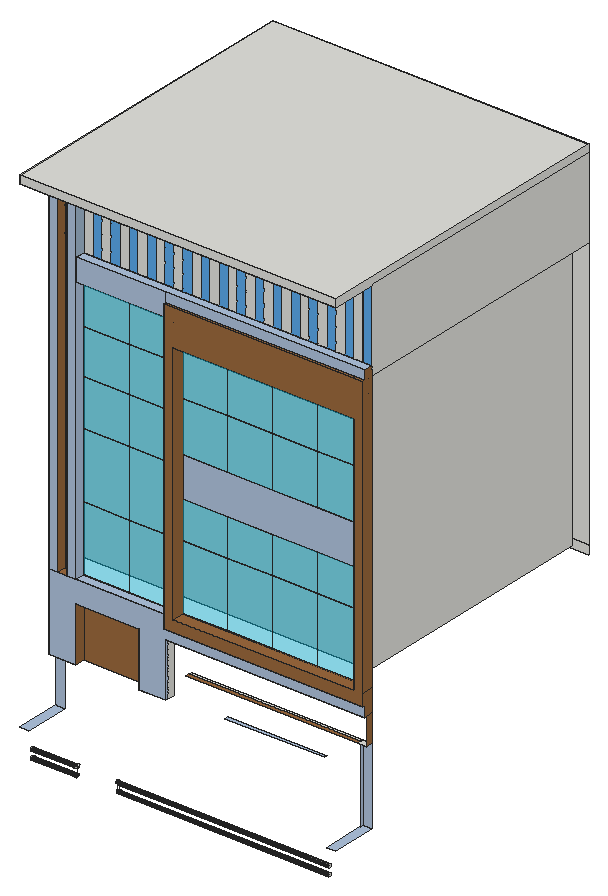
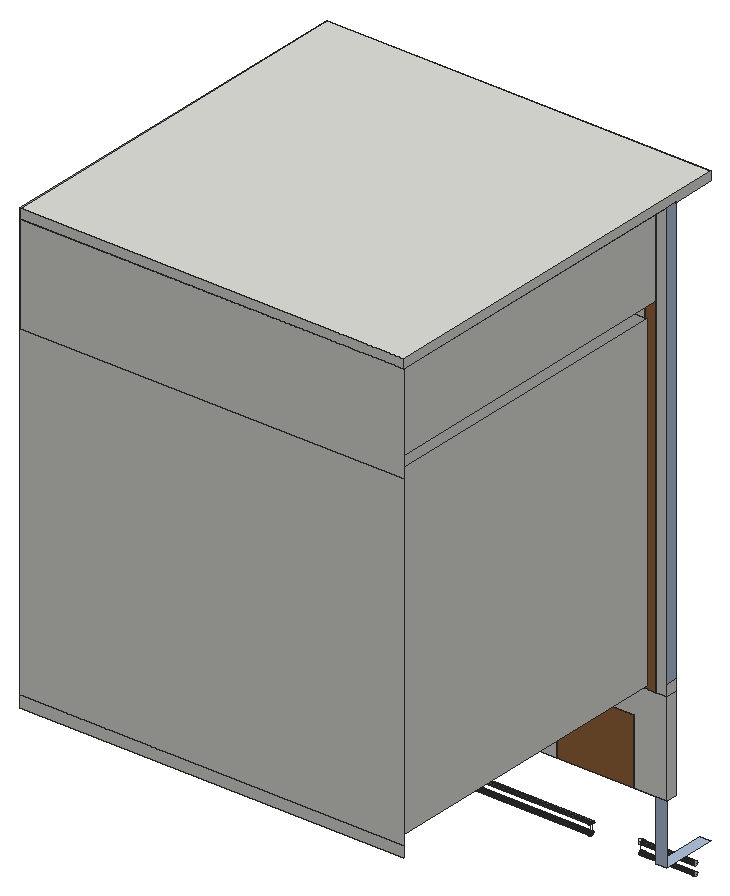
# SketchUp Ruby script. Lengths in inches.
U = 1.inch
M = Sketchup.active_model
def pt(a) = Geom::Point3d.new(a.map { |v| v * U })
def face(e, loops, mat)
  f = e.add_face(loops[0].map { |a| pt(a) })
  loops[1..].each { |l| e.add_face(l.map { |a| pt(a) }).erase! }
  f.material = f.back_material = mat if mat
  f
end
# faces: each face lists its corners as indices into pts; further lists are holes
def faces(e, pts, list, mat = nil) = list.each { |f| face(e, (f[0].is_a?(Array) ? f : [f]).map { |l| l.map { |i| pts[i] } }, mat) }
# xy, xz, yz: faces in a plane at the given z, y or x. An outline is a flat list of corners, or four numbers for a rectangle; further outlines are holes
def ring(l) = l.size == 4 ? [[l[0], l[1]], [l[2], l[1]], [l[2], l[3]], [l[0], l[3]]] : l.each_slice(2).to_a
def flat(e, list, mat, &to3) = list.each { |f| face(e, (f[0].is_a?(Array) ? f : [f]).map { |l| ring(l).map { |u, v| to3.(u, v) } }, mat) }
def xy(e, z, list, mat = nil) = flat(e, list, mat) { |x, y| [x, y, z] }
def xz(e, y, list, mat = nil) = flat(e, list, mat) { |x, z| [x, y, z] }
def yz(e, x, list, mat = nil) = flat(e, list, mat) { |y, z| [x, y, z] }
def lines(e, pts, list) = list.each { |a, b| e.add_line(pt(pts[a]), pt(pts[b])) }
# prism: a flat outline (further loops are holes) pulled along v
def prism(e, loops, v, mat = nil)
  f = face(e, loops, mat); d = Geom::Vector3d.new(v.map { |x| x * U })
  f.pushpull(f.normal.samedirection?(d) ? d.length : -d.length)
end
def box(e, o, s, mat = nil) = prism(e, [[o, [o[0] + s[0], o[1], o[2]], [o[0] + s[0], o[1] + s[1], o[2]], [o[0], o[1] + s[1], o[2]]]], [0, 0, s[2]], mat)
def at(x, y, z, deg = 0) = Geom::Transformation.translation(pt([x, y, z])) * Geom::Transformation.rotation(ORIGIN, Z_AXIS, deg.degrees)
def axes(o, x, y, z) = Geom::Transformation.new([*x, 0, *y, 0, *z, 0, *pt(o).to_a, 1])
def part(name) = M.definitions.add(name)
# library, detail: a bought-in or finely detailed component or shape, given as its bounding box
def library(name, o, s) = part(name).tap { |d| box(d.entities, o, s) }
def detail(e, o, s) = box(e.add_group.entities, o, s)
def put(e, d, t, mat = nil) = e.add_instance(d, t).tap { |i| i.material = mat if mat }
def group(e, t, mat = nil) = e.add_group.tap { |g| g.transformation = t; g.material = mat if mat }.entities
root = M.entities
M.materials.add("[0099_LightSteelBlue]").color = [176, 196, 222]
M.materials.add("[0100_SteelBlue]").color = [91, 169, 234]
M.materials.add("[0110_LightSlateGray]").color = [164, 188, 211]
M.materials.add("[Metal Corrugated Shiny]").color = [124, 124, 124]
M.materials.add("[Translucent Glass Tinted]").color = [8, 201, 241]
M.materials["[Translucent Glass Tinted]"].alpha = 0.48
M.materials.add("[Wood Floor]").color = [155, 105, 61]
xy(root,151.31,[[126.03,62.85,126.54,62.97,126.99,63.22,127.37,63.58,127.64,64.02,127.79,64.52,127.8,64.83,127.8,65.05,127.68,65.55,127.43,66.01,127.07,66.39,126.625,66.66,126.125,66.81,125.6,66.82,125.1,66.7,124.64,66.45,124.26,66.09,123.99,65.64,123.84,65.14,123.83,64.62,123.95,64.11,124.2,63.66,124.56,63.28,125.01,63.01,125.51,62.86]])
xy(root,153,[[72.44,62.83,72.96,62.9,73.44,63.1,73.86,63.42,74.17,63.83,74.375,64.32,74.44,64.83,74.375,65.35,74.17,65.83,73.86,66.25,73.44,66.57,72.96,66.77,72.44,66.83,71.92,66.77,71.44,66.57,71.03,66.25,70.71,65.83,70.51,65.35,70.44,64.83,70.51,64.32,70.71,63.83,71.03,63.42,71.44,63.1,71.92,62.9]])
xy(root,175,[[0,60,12,120],[408,60,420,120]],"[0099_LightSteelBlue]")
xy(root,241,[[0,108,12,120],[12,108,36,120],[120,108,156,120],[228,116,360,120]],"[0099_LightSteelBlue]")
xy(root,277,[[408,111,420,120],[180,116,408,120]])
xy(root,277,[[180,111,408,116]],"[Wood Floor]")
xy(root,313,[[156,111,420,120]])
xy(root,313,[[156,108,420,111]],"[0099_LightSteelBlue]")
xy(root,313,[[36,108,120,120]],"[Wood Floor]")
xy(root,328,[[156,104,420,108]],"[Wood Floor]")
xy(root,343,[[167.5,104,168,108],[408,104,420,120],[0,108,12,120],[24,108,36,120],[167.5,108,168,120]])
xy(root,343,[[36,108,167.5,120]],"[0099_LightSteelBlue]")
xy(root,343,[[168,104,408,120],[12,108,24,120]],"[Wood Floor]")
xy(root,355,[[12,132,408,468]])
xy(root,667,[[167.5,104,168,108],[156,108,167.5,120],[167.5,108,168,120],[201.43,110.45,200.65,110.5,199.91,110.76,199.26,111.2,198.75,111.79,198.41,112.5,198.26,113.27,198.32,114.05,198.58,114.79,199.02,115.44,199.61,115.95,200.3125,116.29,201.08,116.4375,201.86,116.38,202.6,116.12,203.25,115.68,203.76,115.09,204.11,114.39,204.25,113.62,204.2,112.84,203.9375,112.1,203.5,111.45,202.91,110.94,202.2,110.59],[261.5,110.45,260.71,110.5,259.97,110.76,259.33,111.2,258.8125,111.79,258.47,112.5,258.33,113.27,258.38,114.05,258.64,114.79,259.08,115.44,259.67,115.95,260.375,116.29,261.15,116.4375,261.93,116.38,262.67,116.12,263.3125,115.68,263.83,115.09,264.17,114.39,264.32,113.62,264.26,112.84,264,112.1,263.5625,111.45,262.97,110.94,262.26,110.59],
  [323.56,110.45,322.78,110.5,322.04,110.76,321.39,111.2,320.875,111.79,320.54,112.5,320.39,113.27,320.44,114.05,320.7,114.79,321.14,115.44,321.73,115.95,322.4375,116.29,323.21,116.4375,323.99,116.38,324.73,116.12,325.375,115.68,325.89,115.09,326.23,114.39,326.38,113.62,326.32,112.84,326.0625,112.1,325.625,111.45,325.03,110.94,324.33,110.59],[380.12,110.45,379.34,110.5,378.6,110.76,377.95,111.2,377.4375,111.79,377.1,112.5,376.95,113.27,377.01,114.05,377.26,114.79,377.7,115.44,378.3,115.95,379,116.29,379.77,116.4375,380.55,116.38,381.29,116.12,381.9375,115.68,382.45,115.09,382.79,114.39,382.94,113.62,382.88,112.84,382.625,112.1,382.1875,111.45,381.59,110.94,380.89,110.59]])
xy(root,667,[[[168,104,408,120],[261.5,110.45,262.26,110.59,262.97,110.94,263.5625,111.45,264,112.1,264.26,112.84,264.32,113.62,264.17,114.39,263.83,115.09,263.3125,115.68,262.67,116.12,261.93,116.38,261.15,116.4375,260.375,116.29,259.67,115.95,259.08,115.44,258.64,114.79,258.38,114.05,258.33,113.27,258.47,112.5,258.8125,111.79,259.33,111.2,259.97,110.76,260.71,110.5],[323.56,110.45,324.33,110.59,325.03,110.94,325.625,111.45,326.0625,112.1,326.32,112.84,326.38,113.62,326.23,114.39,325.89,115.09,325.375,115.68,324.73,116.12,323.99,116.38,323.21,116.4375,322.4375,116.29,321.73,115.95,321.14,115.44,320.7,114.79,320.44,114.05,320.39,113.27,320.54,112.5,320.875,111.79,321.39,111.2,322.04,110.76,322.78,110.5],[380.12,110.45,380.89,110.59,381.59,110.94,382.1875,111.45,382.625,112.1,382.88,112.84,382.94,113.62,382.79,114.39,382.45,115.09,381.9375,115.68,381.29,116.12,380.55,116.38,379.77,116.4375,379,116.29,378.3,115.95,377.7,115.44,377.26,114.79,377.01,114.05,376.95,113.27,377.1,112.5,377.4375,111.79,377.95,111.2,378.6,110.76,379.34,110.5],[201.43,110.45,202.2,110.59,202.91,110.94,203.5,111.45,203.9375,112.1,204.2,112.84,204.25,113.62,204.11,114.39,203.76,115.09,203.25,115.68,202.6,116.12,201.86,116.38,201.08,116.4375,200.3125,116.29,199.61,115.95,199.02,115.44,198.58,114.79,198.32,114.05,198.26,113.27,198.41,112.5,198.75,111.79,199.26,111.2,199.91,110.76,200.65,110.5]]],"[Wood Floor]")
xy(root,697,[[36,108,156,120],[156,108,168,120]])
xy(root,715,[[156,104,408,108],[408,104,420,108]],"[Wood Floor]")
xy(root,727,[[36,108,420,120]],"[0099_LightSteelBlue]")
xy(root,822.5,[[12,120,408,468]])
xy(root,822.6875,[[82.7,87.46,81.41,87.61,80.2,88.1,79.15,88.88,78.34,89.91,77.83,91.11,77.64,92.4,77.8,93.69,78.28,94.91,79.0625,95.95,80.09,96.76,81.29,97.27,82.58,97.46,83.875,97.3,85.09,96.82,86.13,96.04,86.94,95.01,87.46,93.8125,87.64,92.52,87.49,91.23,87,90.01,86.22,88.97,85.2,88.16,84,87.65],[149.39,87.46,148.1,87.61,146.88,88.1,145.84,88.88,145.03,89.91,144.52,91.11,144.33,92.4,144.48,93.69,144.97,94.91,145.75,95.95,146.78,96.76,147.98,97.27,149.27,97.46,150.5625,97.3,151.78,96.82,152.82,96.04,153.63,95.01,154.14,93.8125,154.33,92.52,154.17,91.23,153.69,90.01,152.91,88.97,151.88,88.16,150.68,87.65],[227.64,87.46,226.35,87.61,225.13,88.1,224.09,88.88,223.28,89.91,222.77,91.11,222.58,92.4,222.73,93.69,223.22,94.91,224,95.95,225.03,96.76,226.23,97.27,227.52,97.46,228.8125,97.3,230.03,96.82,231.07,96.04,231.88,95.01,232.39,93.8125,232.58,92.52,232.42,91.23,231.94,90.01,231.16,88.97,230.13,88.16,228.93,87.65],[312.95,87.46,311.66,87.61,310.45,88.1,309.4,88.88,308.59,89.91,308.08,91.11,307.89,92.4,308.05,93.69,308.53,94.91,309.3125,95.95,310.34,96.76,311.54,97.27,312.83,97.46,314.125,97.3,315.34,96.82,316.38,96.04,317.19,95.01,317.71,93.8125,317.89,92.52,317.74,91.23,317.25,90.01,316.47,88.97,315.45,88.16,314.25,87.65]])
xy(root,822.6875,[[[0,60,0,108,12,108,12,120,24,120,24,108,36,108,36,120,420,120,420,60],[312.95,87.46,314.25,87.65,315.45,88.16,316.47,88.97,317.25,90.01,317.74,91.23,317.89,92.52,317.71,93.8125,317.19,95.01,316.38,96.04,315.34,96.82,314.125,97.3,312.83,97.46,311.54,97.27,310.34,96.76,309.3125,95.95,308.53,94.91,308.05,93.69,307.89,92.4,308.08,91.11,308.59,89.91,309.4,88.88,310.45,88.1,311.66,87.61],[149.39,87.46,150.68,87.65,151.88,88.16,152.91,88.97,153.69,90.01,154.17,91.23,154.33,92.52,154.14,93.8125,153.63,95.01,152.82,96.04,151.78,96.82,150.5625,97.3,149.27,97.46,147.98,97.27,146.78,96.76,145.75,95.95,144.97,94.91,144.48,93.69,144.33,92.4,144.52,91.11,145.03,89.91,145.84,88.88,146.88,88.1,148.1,87.61],[227.64,87.46,228.93,87.65,230.13,88.16,231.16,88.97,231.94,90.01,232.42,91.23,232.58,92.52,232.39,93.8125,231.88,95.01,231.07,96.04,230.03,96.82,228.8125,97.3,227.52,97.46,226.23,97.27,225.03,96.76,224,95.95,223.22,94.91,222.73,93.69,222.58,92.4,222.77,91.11,223.28,89.91,224.09,88.88,225.13,88.1,226.35,87.61],[82.7,87.46,84,87.65,85.2,88.16,86.22,88.97,87,90.01,87.49,91.23,87.64,92.52,87.46,93.8125,86.94,95.01,86.13,96.04,85.09,96.82,83.875,97.3,82.58,97.46,81.29,97.27,80.09,96.76,79.0625,95.95,78.28,94.91,77.8,93.69,77.64,92.4,77.83,91.11,78.34,89.91,79.15,88.88,80.2,88.1,81.41,87.61]]],"[0100_SteelBlue]")
xy(root,823,[[0,108,12,120],[24,108,36,120],[0,120,0,480,420,480,420,120,408,120,408,468,12,468,12,120],[12,120,408,468]])
xy(root,833,[[0,60,420,480]])
xz(root,60,[[0,822.6875,420,833]])
xz(root,104,[[156,328,420,328,420,343,167.5,343,167.5,667,408,667,408,343,420,343,420,715,156,715],[167.5,343,168,667]],"[Wood Floor]")
xz(root,108,[[156,667,168,697],[0,822.6875,12,823],[24,822.6875,36,823]])
xz(root,108,[[0,241,36,241,36,313,120,313,120,241,156,241,156,313,420,313,420,328,156,328,156,343,0,343],[0,343,12,822.6875],[24,343,36,822.6875],[36,697,156,727],[156,715,420,727]],"[0099_LightSteelBlue]")
xz(root,120,[[0,241,0,343,420,343,420,313,156,313,156,241,120,241,120,313,36,313,36,241],[0,343,12,823],[24,343,36,727],[167.5,343,168,667],[408,343,420,355],
  [408,355,420,697],[168,667,168,697,36,697,36,727,420,727,420,697,408,697,408,667],[156,667,168,697],[24,727,36,822.5],[36,727,48,822.5],
  [60,727,72,822.5],[84,727,96,822.5],[108,727,120,822.5],[132,727,144,822.5],[156,727,168,822.5],
  [180,727,192,822.5],[204,727,216,822.5],[228,727,240,822.5],[252,727,264,822.5],[276,727,288,822.5],
  [300,727,312,822.5],[324,727,336,822.5],[348,727,360,822.5],[372,727,384,822.5],[396,727,408,822.5],
  [12,822.5,24,822.6875],[24,822.5,36,823],[36,822.5,48,822.6875],[48,822.5,60,822.6875],[60,822.5,72,822.6875],
  [72,822.5,84,822.6875],[84,822.5,96,822.6875],[96,822.5,108,822.6875],[108,822.5,120,822.6875],[120,822.5,132,822.6875],
  [132,822.5,144,822.6875],[144,822.5,156,822.6875],[156,822.5,168,822.6875],[168,822.5,180,822.6875],[180,822.5,192,822.6875],
  [192,822.5,204,822.6875],[204,822.5,216,822.6875],[216,822.5,228,822.6875],[228,822.5,240,822.6875],[240,822.5,252,822.6875],
  [252,822.5,264,822.6875],[264,822.5,276,822.6875],[276,822.5,288,822.6875],[288,822.5,300,822.6875],[300,822.5,312,822.6875],
  [312,822.5,324,822.6875],[324,822.5,336,822.6875],[336,822.5,348,822.6875],[348,822.5,360,822.6875],[360,822.5,372,822.6875],
  [372,822.5,384,822.6875],[384,822.5,396,822.6875],[396,822.5,408,822.6875],[12,822.6875,24,823],[36,822.6875,48,823],
  [48,822.6875,60,823],[60,822.6875,72,823],[72,822.6875,84,823],[84,822.6875,96,823],[96,822.6875,108,823],
  [108,822.6875,120,823],[120,822.6875,132,823],[132,822.6875,144,823],[144,822.6875,156,823],[156,822.6875,168,823],
  [168,822.6875,180,823],[180,822.6875,192,823],[192,822.6875,204,823],[204,822.6875,216,823],[216,822.6875,228,823],
  [228,822.6875,240,823],[240,822.6875,252,823],[252,822.6875,264,823],[264,822.6875,276,823],[276,822.6875,288,823],
  [288,822.6875,300,823],[300,822.6875,312,823],[312,822.6875,324,823],[324,822.6875,336,823],[336,822.6875,348,823],
  [348,822.6875,360,823],[360,822.6875,372,823],[372,822.6875,384,823],[384,822.6875,396,823],[396,822.6875,408,823],
  [408,822.6875,420,823]])
xz(root,120,[[0,175,12,241],[408,175,420,277],[168,479.27,408,531.9]],"[0099_LightSteelBlue]")
xz(root,120,[[48,727,60,822.5],[72,727,84,822.5],[96,727,108,822.5],[120,727,132,822.5],[144,727,156,822.5],
  [168,727,180,822.5],[192,727,204,822.5],[216,727,228,822.5],[240,727,252,822.5],[264,727,276,822.5],
  [288,727,300,822.5],[312,727,324,822.5],[336,727,348,822.5],[360,727,372,822.5],[384,727,396,822.5],
  [408,727,420,822.6875]],"[0100_SteelBlue]")
xz(root,120,[[36,343,98.3125,429.625],[98.3125,343,167.5,429.625],[168,343,228,429.625],[228,343,288,429.625],[288,343,348,429.625],
  [348,343,408,429.625],[36,429.625,98.3125,516.6875],[98.3125,429.625,167.5,516.6875],[168,429.625,228,479.27],[228,429.625,288,479.27],
  [288,429.625,348,479.27],[348,429.625,408,479.27],[36,516.6875,98.3125,578.8125],[98.3125,516.6875,167.5,578.8125],[168,531.9,228,599.25],
  [228,531.9,288,599.25],[288,531.9,348,599.25],[348,531.9,408,599.25],[36,578.8125,98.3125,638.75],[98.3125,578.8125,167.5,638.75],
  [168,599.25,228,667],[228,599.25,288,667],[288,599.25,348,667],[348,599.25,408,667],[36,638.75,98.3125,697],
  [98.3125,638.75,167.5,638.75,167.5,667,156,667,156,697,98.3125,697]],"[Translucent Glass Tinted]")
xz(root,120,[[36,241,120,313],[12,343,24,822.5]],"[Wood Floor]")
xz(root,132,[[12,355,408,715]])
xz(root,468,[[12,355,408,715],[12,727,408,822.5],[12,822.5,408,823]])
xz(root,480,[[0,343,420,355],[0,355,420,715],[0,715,420,823],[0,823,420,833]])
yz(root,0,[[108,241,120,343],[108,343,120,355],[60,822.6875,60,833,480,833,480,823,108,823,108,822.6875]])
yz(root,0,[[108,355,120,823]],"[0099_LightSteelBlue]")
yz(root,12,[[64.83,138.5625,64.32,138.63,63.83,138.83,63.42,139.15,63.1,139.5625,62.9,140.05,62.83,140.5625,62.9,141.08,63.1,141.5625,63.42,141.98,63.83,142.3,64.32,142.5,64.83,142.5625,65.35,142.5,65.83,142.3,66.25,141.98,66.57,141.5625,66.77,141.08,66.83,140.5625,66.77,140.05,66.57,139.5625,66.25,139.15,65.83,138.83,65.35,138.63],[64.83,149.25,64.32,149.32,63.83,149.52,63.42,149.84,63.1,150.25,62.9,150.73,62.83,151.25,62.9,151.77,63.1,152.25,63.42,152.67,63.83,152.98,64.32,153.18,64.83,153.25,65.35,153.18,65.83,152.98,66.25,152.67,66.57,152.25,66.77,151.77,66.83,151.25,66.77,150.73,66.57,150.25,66.25,149.84,65.83,149.52,65.35,149.32],[132,355,468,715],[120,727,468,822.5],[120,822.5,468,823],
  [108,822.6875,120,823]])
yz(root,12,[[108,343,120,822.6875]],"[Wood Floor]")
yz(root,24,[[108,822.6875,120,823]])
yz(root,24,[[108,343,120,822.6875]],"[Wood Floor]")
yz(root,36,[[108,697,120,727],[108,822.6875,120,823]])
yz(root,36,[[108,343,120,697]],"[0099_LightSteelBlue]")
yz(root,36,[[108,727,120,822.6875]],"[0110_LightSlateGray]")
yz(root,36,[[108,241,120,313]],"[Wood Floor]")
yz(root,70.8125,[[64.83,149.25,65.35,149.32,65.83,149.52,66.25,149.84,66.57,150.25,66.77,150.73,66.83,151.25,66.77,151.77,66.57,152.25,66.25,152.67,65.83,152.98,65.35,153.18,64.83,153.25,64.32,153.18,63.83,152.98,63.42,152.67,63.1,152.25,62.9,151.77,62.83,151.25,62.9,150.73,63.1,150.25,63.42,149.84,63.83,149.52,64.32,149.32]])
yz(root,74.44,[[64.83,151.26,64.84,151.27,64.83,151.27]],"[Metal Corrugated Shiny]")
yz(root,120,[[108,241,120,313]],"[Wood Floor]")
yz(root,156,[[111,241,120,313],[104,328,108,343],[108,667,120,697]])
yz(root,156,[[108,241,111,313]],"[0099_LightSteelBlue]")
yz(root,156,[[104,343,108,697],[104,697,108,715]],"[Wood Floor]")
yz(root,167.5,[[104,343,120,667]],"[Wood Floor]")
yz(root,168,[[108,667,120,697]])
yz(root,168,[[104,343,120,667]],"[Wood Floor]")
yz(root,408,[[64.83,138.5625,65.35,138.63,65.83,138.83,66.25,139.15,66.57,139.5625,66.77,140.05,66.83,140.5625,66.77,141.08,66.57,141.5625,66.25,141.98,65.83,142.3,65.35,142.5,64.83,142.5625,64.32,142.5,63.83,142.3,63.42,141.98,63.1,141.5625,62.9,141.08,62.83,140.5625,62.9,140.05,63.1,139.5625,63.42,139.15,63.83,138.83,64.32,138.63],[64.83,149.25,65.35,149.32,65.83,149.52,66.25,149.84,66.57,150.25,66.77,150.73,66.83,151.25,66.77,151.77,66.57,152.25,66.25,152.67,65.83,152.98,65.35,153.18,64.83,153.25,64.32,153.18,63.83,152.98,63.42,152.67,63.1,152.25,62.9,151.77,62.83,151.25,62.9,150.73,63.1,150.25,63.42,149.84,63.83,149.52,64.32,149.32],[132,355,468,715],[114,667,120,697],[120,727,468,822.5],
  [120,822.5,468,823]])
yz(root,408,[[116,175,120,277]],"[0099_LightSteelBlue]")
yz(root,408,[[104,343,120,667]],"[Wood Floor]")
yz(root,420,[[120,715,480,823],[60,822.6875,120,822.6875,120,823,480,823,480,833,60,833]])
yz(root,420,[[111,277,120,313],[108,313,120,313,120,343,104,343,104,328,108,328],[104,343,120,343,120,727,108,727,108,715,104,715]],"[Wood Floor]")
p = [[12,63.83,138.83],[12,64.32,138.63],[70.51,64.32,138.63],[72.44,64.32,138.63],[72.44,63.83,138.83],[70.71,63.83,138.83],
  [408,64.32,138.63],[408,63.83,138.83],[125.82,63.83,138.83],[125.82,64.32,138.63],[12,64.83,138.5625],[70.44,64.83,138.5625],
  [72.44,64.83,138.5625],[408,64.83,138.5625],[125.82,64.83,138.5625],[127.8,64.83,138.5625],[12,65.35,138.63],[70.51,65.35,138.63],
  [72.44,65.35,138.63],[408,65.35,138.63],[125.82,65.35,138.63],[12,65.83,138.83],[70.71,65.83,138.83],[72.44,65.83,138.83],
  [408,65.83,138.83],[125.82,65.83,138.83],[12,63.42,139.15],[72.44,63.42,139.15],[71.03,63.42,139.15],[408,63.42,139.15],
  [125.82,63.42,139.15],[12,66.25,139.15],[71.03,66.25,139.15],[72.44,66.25,139.15],[408,66.25,139.15],[125.82,66.25,139.15],
  [12,63.1,139.5625],[72.44,63.1,139.5625],[71.44,63.1,139.5625],[408,63.1,139.5625],[125.82,63.1,139.5625],[12,66.57,139.5625],
  [71.44,66.57,139.5625],[72.44,66.57,139.5625],[408,66.57,139.5625],[125.82,66.57,139.5625],[12,62.9,140.05],[72.44,62.9,140.05],
  [71.92,62.9,140.05],[408,62.9,140.05],[125.82,62.9,140.05],[12,66.77,140.05],[71.92,66.77,140.05],[72.44,66.77,140.05],
  [408,66.77,140.05],[125.82,66.77,140.05],[12,62.83,140.5625],[72.44,62.83,140.5625],[408,62.83,140.5625],[125.82,62.83,140.5625],
  [12,66.83,140.5625],[72.44,66.83,140.5625],[408,66.83,140.5625],[125.82,66.83,140.5625],[12,62.9,141.08],[72.44,62.9,141.08],
  [71.92,62.9,141.08],[408,62.9,141.08],[125.82,62.9,141.08],[12,66.77,141.08],[71.92,66.77,141.08],[72.44,66.77,141.08],
  [408,66.77,141.08],[125.82,66.77,141.08],[12,63.1,141.5625],[72.44,63.1,141.5625],[71.44,63.1,141.5625],[408,63.1,141.5625],
  [125.82,63.1,141.5625],[12,66.57,141.5625],[71.44,66.57,141.5625],[72.44,66.57,141.5625],[408,66.57,141.5625],[125.82,66.57,141.5625],
  [12,63.42,141.98],[72.44,63.42,141.98],[71.03,63.42,141.98],[408,63.42,141.98],[125.82,63.42,141.98],[12,66.25,141.98],
  [71.03,66.25,141.98],[72.44,66.25,141.98],[408,66.25,141.98],[125.82,66.25,141.98],[12,63.83,142.3],[72.44,63.83,142.3],
  [70.71,63.83,142.3],[408,63.83,142.3],[125.82,63.83,142.3],[12,65.83,142.3],[70.71,65.83,142.3],[72.44,65.83,142.3],
  [408,65.83,142.3],[125.82,65.83,142.3],[12,64.32,142.5],[72.44,64.32,142.5],[70.51,64.32,142.5],[408,64.32,142.5],
  [125.82,64.32,142.5],[12,65.35,142.5],[70.51,65.35,142.5],[72.44,65.35,142.5],[408,65.35,142.5],[125.82,65.35,142.5],
  [12,64.83,142.5625],[72.44,64.83,142.5625],[70.44,64.83,142.5625],[408,64.83,142.5625],[127.8,64.83,142.5625],[125.82,64.83,142.5625],
  [12,63.83,149.52],[12,64.32,149.32],[70.51,64.32,149.32],[70.8125,64.32,149.32],[70.8125,63.83,149.52],[70.71,63.83,149.52],
  [408,64.32,149.32],[408,63.83,149.52],[127.83,63.83,149.52],[127.65,64.32,149.32],[12,64.83,149.25],[70.44,64.83,149.25],
  [70.8125,64.83,149.25],[408,64.83,149.25],[127.33,64.83,149.25],[127.8,64.83,149.25],[12,65.35,149.32],[70.51,65.35,149.32],
  [70.8125,65.35,149.32],[408,65.35,149.32],[126.92,65.35,149.32],[12,65.83,149.52],[70.71,65.83,149.52],[70.8125,65.83,149.52],
  [408,65.83,149.52],[126.43,65.83,149.52],[12,63.42,149.84],[70.8125,63.42,149.84],[408,63.42,149.84],[127.88,63.42,149.84],
  [12,66.25,149.84],[70.8125,66.25,149.84],[408,66.25,149.84],[125.9,66.25,149.84],[12,63.1,150.25],[70.8125,63.1,150.25],
  [408,63.1,150.25],[127.79,63.1,150.25],[12,66.57,150.25],[70.8125,66.57,150.25],[408,66.57,150.25],[125.36,66.57,150.25],
  [73.45,66.12,150.09],[72.96,66.26,149.95],[72.45,66.31,149.9],[71.93,66.26,149.95],[71.45,66.11,150.08],[71.03,65.875,150.29],
  [70.71,65.57,150.57],[70.51,65.21,150.89],[70.44,64.83,151.23],[70.44,64.83,151.24],[70.51,64.45,151.59],[70.71,64.09,151.91],
  [71.02,63.79,152.2],[71.4375,63.55,152.41],[71.92,63.41,152.55],[72.4375,63.36,152.6],[72.95,63.41,152.56],[73.4375,63.56,152.43],
  [73.85,63.79,152.22],[74.17,64.1,151.9375],[74.37,64.46,151.61],[74.44,64.83,151.27],[74.44,64.84,151.27],[74.375,65.22,150.92],
  [74.18,65.58,150.59],[73.86,65.88,150.31],[12,62.9,150.73],[70.8125,62.9,150.73],[408,62.9,150.73],[127.57,62.9,150.73],
  [12,66.77,150.73],[70.8125,66.77,150.73],[408,66.77,150.73],[124.85,66.77,150.73],[12,62.83,151.25],[70.8125,62.83,151.25],
  [408,62.83,151.25],[127.22,62.83,151.25],[12,66.83,151.25],[70.8125,66.83,151.25],[408,66.83,151.25],[124.41,66.83,151.25],
  [12,62.9,151.77],[70.8125,62.9,151.77],[408,62.9,151.77],[126.78,62.9,151.77],[12,66.77,151.77],[70.8125,66.77,151.77],
  [408,66.77,151.77],[124.07,66.77,151.77],[12,63.1,152.25],[70.8125,63.1,152.25],[408,63.1,152.25],[126.27,63.1,152.25],
  [12,66.57,152.25],[70.8125,66.57,152.25],[408,66.57,152.25],[123.84,66.57,152.25],[12,63.42,152.67],[70.8125,63.42,152.67],
  [408,63.42,152.67],[125.74,63.42,152.67],[12,66.25,152.67],[70.8125,66.25,152.67],[408,66.25,152.67],[123.75,66.25,152.67],
  [12,63.83,152.98],[70.8125,63.83,152.98],[70.71,63.83,152.98],[408,63.83,152.98],[125.2,63.83,152.98],[12,65.83,152.98],
  [70.71,65.83,152.98],[70.8125,65.83,152.98],[408,65.83,152.98],[123.8,65.83,152.98],[12,64.32,153.18],[70.8125,64.32,153.18],
  [408,64.32,153.18],[124.71,64.32,153.18],[12,65.35,153.18],[70.8125,65.35,153.18],[408,65.35,153.18],[123.99,65.35,153.18],
  [12,64.83,153.25],[70.8125,64.83,153.25],[408,64.83,153.25],[124.3,64.83,153.25],[408,114,715],[408,114,697],
  [420,114,715],[420,114,697],[408,108,715],[168,108,697],[168,104,697],[156,108,670],
  [167.5,104,667],[408,132.49,727],[408,132.49,715],[12,64.83,151.25],[70.44,64.83,151.25],[70.8125,64.83,151.25],
  [72.44,64.83,151.25],[12,64.83,140.5625],[70.44,64.83,140.5625],[408,64.83,140.5625],[127.8,64.83,140.5625],[408,64.83,151.25],
  [127.8,64.83,151.25],[125.82,64.83,151.25],[72.44,64.83,140.5625],[125.82,64.83,140.5625],[127.8,64.83,151.31]]
faces(root,p,[[0,1,2,3,4,5],[6,7,8,9],[1,10,11,12,3,2],[13,6,9,14,15],[10,16,17,18,12,11],[19,13,15,14,20],[16,21,22,23,18,17],[24,19,20,25],
  [26,0,5,4,27,28],[7,29,30,8],[21,31,32,33,23,22],[34,24,25,35],[36,26,28,27,37,38],[29,39,40,30],[31,41,42,43,33,32],[44,34,35,45],
  [46,36,38,37,47,48],[39,49,50,40],[41,51,52,53,43,42],[54,44,45,55],[56,46,48,47,57],[49,58,59,50],[51,60,61,53,52],[62,54,55,63],
  [64,56,57,65,66],[58,67,68,59],[60,69,70,71,61],[72,62,63,73],[74,64,66,65,75,76],[67,77,78,68],[69,79,80,81,71,70],[82,72,73,83],
  [84,74,76,75,85,86],[77,87,88,78],[79,89,90,91,81,80],[92,82,83,93],[94,84,86,85,95,96],[87,97,98,88],[89,99,100,101,91,90],[102,92,93,103],
  [104,94,96,95,105,106],[97,107,108,98],[99,109,110,111,101,100],[112,102,103,113],[114,104,106,105,115,116],[107,117,118,119,108],[109,114,116,115,111,110],[117,112,113,119,118],
  [120,121,122,123,124,125],[126,127,128,129],[121,130,131,132,123,122],[133,126,129,134,135],[130,136,137,138,132,131],[139,133,135,134,140],[136,141,142,143,138,137],[144,139,140,145],
  [146,120,125,124,147],[127,148,149,128],[141,150,151,143,142],[152,144,145,153],[154,146,147,155],[148,156,157,149],[150,158,159,151],[160,152,153,161],
  [188,154,155,189],[156,190,191,157],[158,192,193,159],[194,160,161,195],[196,188,189,197],[190,198,199,191],[192,200,201,193],[202,194,195,203],
  [204,196,197,205],[198,206,207,199],[200,208,209,201],[210,202,203,211],[212,204,205,213],[206,214,215,207],[208,216,217,209],[218,210,211,219],
  [220,212,213,221],[214,222,223,215],[216,224,225,217],[226,218,219,227],[228,220,221,229,230],[222,231,232,223],[224,233,234,235,225],[236,226,227,237],
  [238,228,230,229,239],[231,240,241,232],[233,242,243,235,234],[244,236,237,245],[246,238,239,247],[240,248,249,241],[242,246,247,243],[248,244,245,249]],"[Metal Corrugated Shiny]")
faces(root,p,[[162,163,164,165,166,167,168,169,170,171,172,173,174,175,176,177,178,179,180,181,182,183,184,185,186,187]])
lines(root,p,[[250,251],[250,252],[251,253],[250,254],[255,256],[257,258],[259,260],[261,262],[263,264],[264,115],[265,266],[267,268],
  [269,270],[119,271],[262,263],[266,272],[268,273],[270,271],[15,268],[268,118],[118,135],[135,270],[270,274]])
